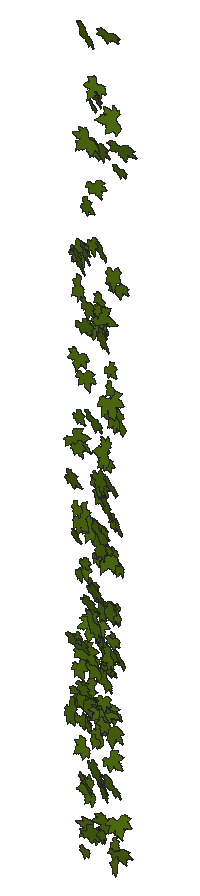
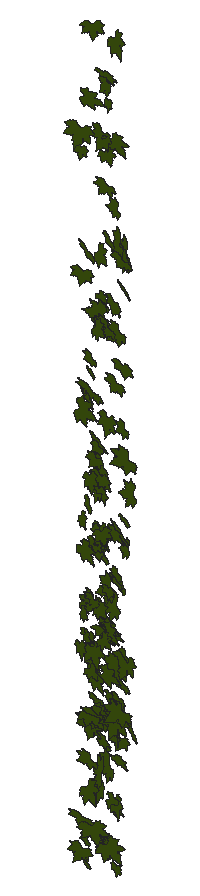
# SketchUp Ruby script. Lengths in inches.
U = 1.inch
M = Sketchup.active_model
def pt(a) = Geom::Point3d.new(a.map { |v| v * U })
def face(e, loops, mat)
  f = e.add_face(loops[0].map { |a| pt(a) })
  loops[1..].each { |l| e.add_face(l.map { |a| pt(a) }).erase! }
  f.material = f.back_material = mat if mat
  f
end
# faces: each face lists its corners as indices into pts; further lists are holes
def faces(e, pts, list, mat = nil) = list.each { |f| face(e, (f[0].is_a?(Array) ? f : [f]).map { |l| l.map { |i| pts[i] } }, mat) }
# xy, xz, yz: faces in a plane at the given z, y or x. An outline is a flat list of corners, or four numbers for a rectangle; further outlines are holes
def ring(l) = l.size == 4 ? [[l[0], l[1]], [l[2], l[1]], [l[2], l[3]], [l[0], l[3]]] : l.each_slice(2).to_a
def flat(e, list, mat, &to3) = list.each { |f| face(e, (f[0].is_a?(Array) ? f : [f]).map { |l| ring(l).map { |u, v| to3.(u, v) } }, mat) }
def xy(e, z, list, mat = nil) = flat(e, list, mat) { |x, y| [x, y, z] }
def xz(e, y, list, mat = nil) = flat(e, list, mat) { |x, z| [x, y, z] }
def yz(e, x, list, mat = nil) = flat(e, list, mat) { |y, z| [x, y, z] }
def lines(e, pts, list) = list.each { |a, b| e.add_line(pt(pts[a]), pt(pts[b])) }
# prism: a flat outline (further loops are holes) pulled along v
def prism(e, loops, v, mat = nil)
  f = face(e, loops, mat); d = Geom::Vector3d.new(v.map { |x| x * U })
  f.pushpull(f.normal.samedirection?(d) ? d.length : -d.length)
end
def box(e, o, s, mat = nil) = prism(e, [[o, [o[0] + s[0], o[1], o[2]], [o[0] + s[0], o[1] + s[1], o[2]], [o[0], o[1] + s[1], o[2]]]], [0, 0, s[2]], mat)
def at(x, y, z, deg = 0) = Geom::Transformation.translation(pt([x, y, z])) * Geom::Transformation.rotation(ORIGIN, Z_AXIS, deg.degrees)
def axes(o, x, y, z) = Geom::Transformation.new([*x, 0, *y, 0, *z, 0, *pt(o).to_a, 1])
def part(name) = M.definitions.add(name)
# library, detail: a bought-in or finely detailed component or shape, given as its bounding box
def library(name, o, s) = part(name).tap { |d| box(d.entities, o, s) }
def detail(e, o, s) = box(e.add_group.entities, o, s)
def put(e, d, t, mat = nil) = e.add_instance(d, t).tap { |i| i.material = mat if mat }
def group(e, t, mat = nil) = e.add_group.tap { |g| g.transformation = t; g.material = mat if mat }.entities
root = M.entities
M.materials.add("[Vegetation Blur 03]").color = [83, 114, 18]
c1 = part("ivy")
xy(c1.entities,0,[[0.782,0,0.786,0,0.787,0.005,0.789,0.009,0.821,0.072,0.875,0.147,1.001,0.272,1.073,0.331,1.137,0.363,1.178,0.379,1.223,0.384,1.272,0.383,1.311,0.374,1.36,0.355,1.399,0.334,1.491,0.285,1.541,0.244,1.583,0.199,1.617,0.15,1.64,0.128,1.662,0.115,1.717,0.105,1.745,0.093,1.784,0.054,1.819,0.057,1.854,0.064,1.882,0.075,1.896,0.074,1.91,0.071,1.937,0.063,1.964,0.053,1.99,0.038,2.016,0.015,2.034,0.002,2.04,0,2.038,0.003,2.036,0.007,2.033,0.038,2.036,0.068,2.045,0.1,2.055,0.116,2.064,0.123,2.077,0.129,2.088,0.129,2.106,0.132,2.118,0.13,2.179,0.132,2.207,0.133,2.225,0.133,2.242,0.138,2.22,0.162,2.207,0.186,2.206,0.213,2.212,0.236,2.228,0.262,2.247,0.274,2.298,0.283,2.355,0.294,2.37,0.296,2.376,0.295,2.377,0.3,2.377,0.303,2.385,0.329,2.411,0.37,2.426,0.392,2.449,0.407,2.511,0.426,2.561,0.444,2.619,0.466,2.589,0.469,2.561,0.476,2.501,0.5,2.449,0.516,2.424,0.523,2.401,0.535,2.377,0.556,2.372,0.568,2.36,0.575,2.268,0.586,2.225,0.592,2.207,0.599,2.194,0.61,2.143,0.65,2.13,0.664,2.122,0.682,2.123,0.7,2.13,0.719,2.148,0.75,2.17,0.781,2.195,0.807,2.221,0.828,2.284,0.874,2.291,0.88,2.288,0.887,2.276,0.9,2.267,0.916,2.265,0.933,2.273,0.967,2.292,1.002,2.313,1.03,2.334,1.054,2.348,1.067,2.358,1.074,2.363,1.076,2.362,1.081,2.35,1.094,2.347,1.11,2.35,1.143,2.359,1.18,2.385,1.254,2.415,1.324,2.448,1.393,2.45,1.4,2.446,1.398,2.44,1.394,2.427,1.383,2.402,1.36,2.376,1.339,2.345,1.324,2.305,1.309,2.282,1.303,2.273,1.306,2.245,1.294,2.212,1.287,2.187,1.291,2.163,1.301,2.142,1.316,2.134,1.327,2.124,1.325,2.09,1.292,2.053,1.259,2.014,1.234,1.973,1.215,1.954,1.21,1.931,1.208,1.909,1.212,1.893,1.22,1.879,1.233,1.872,1.248,1.867,1.281,1.864,1.319,1.821,1.258,1.773,1.197,1.726,1.141,1.698,1.121,1.679,1.116,1.666,1.117,1.647,1.122,1.632,1.129,1.62,1.141,1.617,1.154,1.617,1.219,1.621,1.254,1.623,1.268,1.623,1.281,1.618,1.314,1.606,1.346,1.603,1.375,1.607,1.403,1.603,1.467,1.599,1.499,1.605,1.525,1.614,1.552,1.629,1.577,1.635,1.589,1.629,1.587,1.618,1.582,1.596,1.566,1.581,1.556,1.568,1.552,1.557,1.55,1.545,1.553,1.531,1.562,1.522,1.572,1.504,1.591,1.486,1.611,1.474,1.631,1.457,1.666,1.455,1.684,1.457,1.698,1.452,1.715,1.444,1.728,1.424,1.754,1.419,1.772,1.423,1.786,1.434,1.819,1.444,1.848,1.446,1.855,1.44,1.861,1.43,1.867,1.386,1.904,1.349,1.948,1.326,1.973,1.31,1.995,1.288,2.048,1.284,2.153,1.287,2.254,1.284,2.255,1.282,2.253,1.278,2.247,1.274,2.237,1.266,2.216,1.226,2.125,1.208,2.076,1.184,2.033,1.155,1.984,1.135,1.942,1.111,1.899,1.083,1.861,1.053,1.85,1.059,1.83,1.061,1.809,1.056,1.79,1.049,1.767,1.04,1.749,1.018,1.733,0.994,1.726,0.942,1.734,0.95,1.6875,0.944,1.645,0.932,1.608,0.911,1.585,0.881,1.58,0.854,1.582,0.828,1.588,0.785,1.618,0.773,1.625,0.775,1.614,0.779,1.598,0.796,1.502,0.818,1.402,0.861,1.283,0.882,1.224,0.894,1.174,0.892,1.148,0.886,1.123,0.881,1.107,0.872,1.099,0.849,1.094,0.818,1.092,0.789,1.098,0.762,1.107,0.753,1.113,0.721,1.139,0.698,1.163,0.678,1.194,0.665,1.224,0.628,1.28,0.612,1.312,0.606,1.327,0.606,1.314,0.599,1.282,0.594,1.267,0.581,1.256,0.544,1.245,0.512,1.244,0.473,1.249,0.444,1.256,0.382,1.288,0.339,1.306,0.324,1.316,0.317,1.324,0.309,1.326,0.27,1.314,0.227,1.313,0.185,1.3125,0.152,1.317,0.122,1.328,0.092,1.345,0.073,1.353,0.079,1.338,0.092,1.308,0.117,1.249,0.13,1.215,0.139,1.164,0.147,1.148,0.157,1.136,0.163,1.122,0.174,1.086,0.177,1.067,0.182,1.054,0.186,1.043,0.191,1.038,0.211,1.028,0.237,1.005,0.25,0.974,0.253,0.96,0.25,0.944,0.242,0.914,0.243,0.906,0.249,0.902,0.26,0.894,0.289,0.88,0.307,0.873,0.322,0.862,0.364,0.799,0.403,0.738,0.431,0.709,0.439,0.691,0.441,0.678,0.4375,0.66,0.428,0.645,0.394,0.623,0.303,0.594,0.255,0.581,0.214,0.577,0.179,0.573,0.173,0.568,0.175,0.561,0.167,0.55,0.141,0.523,0.113,0.503,0.077,0.49,0.045,0.486,0.026,0.485,0.019,0.486,0.011,0.483,0,0.471,0.014,0.467,0.044,0.455,0.058,0.447,0.07,0.438,0.097,0.411,0.125,0.394,0.158,0.377,0.174,0.366,0.182,0.359,0.185,0.361,0.242,0.331,0.253,0.316,0.258,0.303,0.262,0.283,0.274,0.278,0.308,0.274,0.341,0.252,0.366,0.226,0.366,0.222,0.37,0.22,0.38,0.221,0.395,0.221,0.425,0.216,0.45,0.207,0.465,0.192,0.473,0.178,0.484,0.15,0.489,0.116,0.483,0.089,0.468,0.058,0.45,0.035,0.435,0.018,0.429,0.011,0.434,0.012,0.438,0.014,0.469,0.019,0.542,0.016,0.581,0.015,0.612,0.027,0.68,0.055,0.696,0.057,0.712,0.052,0.73,0.045,0.741,0.036,0.766,0.014]])
put(root,c1,axes([125.92,173.8,17.01],[0.64437,-0.16461,0.01325],[0.02704,0.17964,-0.52482],[-0.07702,-1.31419,-0.0734]),"[Vegetation Blur 03]")
put(root,c1,axes([125.97,173.8,24.94],[0.20255,-0.18759,0.41357],[0.50926,-0.09194,-0.17269],[-0.07578,-1.11921,-0.05513]),"[Vegetation Blur 03]")
put(root,c1,axes([125.89,173.8,12.75],[0.26152,-0.04302,0.44662],[0.5117,-0.42542,-0.20602],[-0.19512,-1.17335,0.05832]),"[Vegetation Blur 03]")
put(root,c1,axes([125.77,173.8,26.86],[0.3615,0.01419,0.44771],[0.54841,0.02846,-0.29509],[0.01534,-1.35164,-0.00151]),"[Vegetation Blur 03]")
put(root,c1,axes([126.91,173.8,49.39],[0.37946,-0.0754,-0.40939],[-0.47883,0.34147,-0.30552],[-0.15388,-1.24846,-0.05884]),"[Vegetation Blur 03]")
put(root,c1,axes([126.54,173.8,24.12],[0.34373,-0.18323,-0.04475],[-0.06771,-0.09451,-0.28552],[-0.07969,-0.71,0.04955]),"[Vegetation Blur 03]")
put(root,c1,axes([126.41,173.8,16.84],[0.19414,-0.08015,0.20136],[0.24242,-0.09451,-0.1616],[-0.0602,-0.6391,-0.00136]),"[Vegetation Blur 03]")
put(root,c1,axes([126.27,173.8,32.1],[0.54066,-0.11979,-0.01485],[-0.02304,-0.09186,-0.44216],[-0.05647,-1.10941,0.03821]),"[Vegetation Blur 03]")
put(root,c1,axes([126.25,173.8,26.84],[0.30004,-0.03578,0.23182],[0.28092,-0.09842,-0.24458],[-0.04545,-0.84451,0.01868]),"[Vegetation Blur 03]")
put(root,c1,axes([126.29,173.8,12.78],[0.44477,-0.01678,0.0841],[0.10333,0.04659,-0.36253],[-0.00282,-0.93833,-0.0195]),"[Vegetation Blur 03]")
put(root,c1,axes([126.4,173.8,22.17],[0.15681,-0.19135,0.27864],[0.34217,-0.11382,-0.14055],[-0.09017,-0.7647,-0.0488]),"[Vegetation Blur 03]")
put(root,c1,axes([126.36,173.8,28.4375],[0.23733,-0.08095,0.26556],[0.32364,-0.07275,-0.19614],[-0.05179,-0.82556,-0.00876]),"[Vegetation Blur 03]")
put(root,c1,axes([126.15,173.8,37.21],[0.44354,0.00148,0.25414],[0.30752,-0.17731,-0.35733],[-0.04893,-1.101,0.05789]),"[Vegetation Blur 03]")
put(root,c1,axes([126.9,173.8,9.88],[0.41747,-0.18159,-0.28175],[-0.32214,0.27535,-0.34584],[-0.15229,-1.08022,-0.04079]),"[Vegetation Blur 03]")
put(root,c1,axes([126.57,173.8,20.32],[0.21446,-0.11197,0.17329],[0.20462,-0.11686,-0.18055],[-0.07858,-0.60992,0.00278]),"[Vegetation Blur 03]")
put(root,c1,axes([126.19,173.8,37.11],[0.28904,-0.06987,0.39444],[0.46239,-0.30604,-0.23421],[-0.14468,-1.11768,0.03947]),"[Vegetation Blur 03]")
put(root,c1,axes([126.82,173.8,36.16],[0.42016,-0.3703,-0.17602],[-0.23818,-0.04638,-0.36333],[-0.14889,-0.97076,0.0845]),"[Vegetation Blur 03]")
put(root,c1,axes([126.06,173.8,13.94],[0.46309,-0.00814,0.32802],[0.3991,0.15897,-0.37467],[0.04767,-1.25175,-0.04972]),"[Vegetation Blur 03]")
put(root,c1,axes([126.31,173.8,15.31],[0.35031,-0.0224,0.27157],[0.32357,-0.21117,-0.28075],[-0.0784,-0.97156,0.05476]),"[Vegetation Blur 03]")
put(root,c1,axes([127.02,173.8,11.9],[0.35443,-0.19304,-0.2419],[-0.30587,-0.0509,-0.29211],[-0.05567,-0.94941,0.06485]),"[Vegetation Blur 03]")
put(root,c1,axes([126.98,173.8,43.99],[0.532,-0.08529,-0.32199],[-0.3962,-0.04622,-0.4341],[-0.01987,-1.36215,0.03489]),"[Vegetation Blur 03]")
put(root,c1,axes([126.33,173.8,22.68],[0.16553,0.17765,0.51158],[0.60894,-0.40708,-0.109],[-0.17196,-1.2705,0.10646]),"[Vegetation Blur 03]")
put(root,c1,axes([127.1,173.8,13.0625],[0.30175,-0.15566,-0.18852],[-0.22184,0.13329,-0.25383],[-0.09933,-0.77056,-0.00582]),"[Vegetation Blur 03]")
put(root,c1,axes([126.62,173.8,13.79],[0.24227,-0.06001,0.24324],[0.27574,-0.26297,-0.19314],[-0.11679,-0.74533,0.04856]),"[Vegetation Blur 03]")
put(root,c1,axes([127.59,173.8,9.9],[0.23881,-0.20013,-0.4704],[-0.57401,0.16163,-0.20491],[-0.11037,-1.27363,0.04791]),"[Vegetation Blur 03]")
put(root,c1,axes([126.85,173.8,6.07],[0.31854,-0.11206,-0.01065],[-0.01233,0.01101,-0.26373],[-0.05462,-0.65595,-0.00261]),"[Vegetation Blur 03]")
put(root,c1,axes([126.29,173.8,13.81],[0.67064,-0.03297,0.06761],[0.08405,0.14038,-0.54453],[-0.00745,-1.38343,-0.05687]),"[Vegetation Blur 03]")
put(root,c1,axes([126.63,173.8,14.65],[0.43055,-0.17357,0.04955],[0.0586,-0.03425,-0.35804],[-0.08583,-0.8941,0.0041]),"[Vegetation Blur 03]")
put(root,c1,axes([127.21,173.8,7.68],[0.46314,0.05825,-0.39602],[-0.48604,0.04033,-0.37767],[0.00535,-1.37976,-0.02776]),"[Vegetation Blur 03]")
put(root,c1,axes([126.77,173.8,20.93],[0.24085,-0.07286,0.19486],[0.23769,-0.04913,-0.19858],[-0.04198,-0.69616,-0.00638]),"[Vegetation Blur 03]")
put(root,c1,axes([127.5,173.8,23.6875],[0.31165,-0.23246,-0.38206],[-0.4746,0.04633,-0.26229],[-0.08166,-1.15634,0.0663]),"[Vegetation Blur 03]")
put(root,c1,axes([126.45,173.8,33.35],[0.40049,-0.10291,0.28569],[0.35224,0.02026,-0.32774],[-0.03114,-1.09438,-0.03293]),"[Vegetation Blur 03]")
put(root,c1,axes([127.72,173.8,18.65],[0.20411,-0.06117,-0.44075],[-0.53473,0.15542,-0.16833],[-0.08116,-1.17781,0.00068]),"[Vegetation Blur 03]")
put(root,c1,axes([126.75,173.8,20.47],[0.2517,0.01272,0.24338],[0.28699,-0.2291,-0.19581],[-0.08127,-0.76965,0.06231]),"[Vegetation Blur 03]")
put(root,c1,axes([126.33,173.8,37.12],[0.43009,-0.41994,0.38446],[0.46829,-0.19735,-0.38284],[-0.21039,-1.29771,-0.06619]),"[Vegetation Blur 03]")
put(root,c1,axes([126.54,173.8,30.8],[0.46612,-0.06322,0.21313],[0.25778,-0.10592,-0.38046],[-0.05188,-1.09436,0.02451]),"[Vegetation Blur 03]")
put(root,c1,axes([126.33,173.8,15.9375],[0.4004,-0.01607,0.44585],[0.54595,-0.04146,-0.32681],[-0.02086,-1.39316,0.00458]),"[Vegetation Blur 03]")
put(root,c1,axes([127.8,173.8,15.05],[0.07522,-0.13511,-0.31021],[-0.37954,0.11629,-0.06927],[-0.06884,-0.78881,0.04292]),"[Vegetation Blur 03]")
put(root,c1,axes([127.96,173.8,16.33],[0.13923,-0.07198,-0.4584],[-0.56199,0.04465,-0.11479],[-0.02951,-1.18996,0.02342]),"[Vegetation Blur 03]")
put(root,c1,axes([127.37,173.8,43.09],[0.32097,0.04197,-0.19874],[-0.24426,0.07998,-0.2601],[-0.00735,-0.82521,-0.03532]),"[Vegetation Blur 03]")
put(root,c1,axes([126.89,173.8,39.48],[0.11949,-0.05949,0.35767],[0.43416,-0.12523,-0.09989],[-0.06637,-0.92633,-0.00946]),"[Vegetation Blur 03]")
put(root,c1,axes([127.76,173.8,18.05],[0.16976,0.07158,-0.29867],[-0.3654,0.12339,-0.13369],[-0.04012,-0.82092,-0.04613]),"[Vegetation Blur 03]")
put(root,c1,axes([126.89,173.8,34.96],[0.51145,-0.25079,0.06105],[0.06998,-0.0596,-0.42899],[-0.12471,-1.06199,0.00966]),"[Vegetation Blur 03]")
put(root,c1,axes([127.4,173.8,45.46],[0.26677,-0.13263,-0.08131],[-0.08808,0.11667,-0.22242],[-0.07951,-0.57427,-0.02641]),"[Vegetation Blur 03]")
put(root,c1,axes([126.72,173.8,37.63],[0.38011,-0.35457,0.334],[0.40396,-0.18413,-0.33696],[-0.18436,-1.13452,-0.04969]),"[Vegetation Blur 03]")
put(root,c1,axes([127.28,173.8,20.28],[0.33233,-0.0945,-0.02615],[-0.02986,0.03657,-0.27359],[-0.04737,-0.68607,-0.01098]),"[Vegetation Blur 03]")
put(root,c1,axes([128,173.8,38.07],[0.15729,0.04975,-0.38701],[-0.46067,0.26502,-0.11935],[-0.11503,-0.99334,-0.05122]),"[Vegetation Blur 03]")
put(root,c1,axes([127.31,173.8,18.71],[0.56265,-0.26157,-0.25412],[-0.30853,0.09554,-0.47049],[-0.13384,-1.31983,0.01631]),"[Vegetation Blur 03]")
put(root,c1,axes([127.51,173.8,23.48],[0.35115,0.05857,-0.18722],[-0.23024,0.1649,-0.27952],[-0.02054,-0.84722,-0.06735]),"[Vegetation Blur 03]")
put(root,c1,axes([126.87,173.8,6.55],[0.26007,-0.08689,0.38147],[0.46915,0.07766,-0.21026],[0.0126,-1.09796,-0.04506]),"[Vegetation Blur 03]")
put(root,c1,axes([126.98,173.8,18.27],[0.61939,0.05734,-0.0417],[-0.04546,-0.22498,-0.49845],[0.03634,-1.25897,0.08717]),"[Vegetation Blur 03]")
put(root,c1,axes([127.125,173.8,17.87],[0.12985,0.03067,0.35023],[0.42444,-0.14892,-0.10276],[-0.06505,-0.91052,0.02861]),"[Vegetation Blur 03]")
put(root,c1,axes([127.92,173.8,19.54],[0.17674,0.08976,-0.26223],[-0.3229,0.11764,-0.13863],[-0.02967,-0.7454,-0.05345]),"[Vegetation Blur 03]")
put(root,c1,axes([127.11,173.8,29.13],[0.58072,-0.2362,-0.06513],[-0.0644,0.17074,-0.47989],[-0.12408,-1.1941,-0.05574]),"[Vegetation Blur 03]")
put(root,c1,axes([126.87,173.8,18.92],[0.32867,-0.28906,0.36046],[0.45664,0.0115,-0.27589],[-0.07923,-1.13284,-0.09478]),"[Vegetation Blur 03]")
put(root,c1,axes([128.2,173.8,34.0625],[0.08767,0.08949,-0.34433],[-0.41588,0.19217,-0.06267],[-0.08326,-0.86566,-0.04951]),"[Vegetation Blur 03]")
put(root,c1,axes([127.84,173.8,18.08],[0.25432,-0.19046,-0.24423],[-0.28944,0.16036,-0.22043],[-0.11975,-0.79207,0.0141]),"[Vegetation Blur 03]")
put(root,c1,axes([127.08,173.8,40.9],[0.40459,0.02303,0.19859],[0.2435,-0.01333,-0.3302],[0.00625,-0.97145,0.00924]),"[Vegetation Blur 03]")
put(root,c1,axes([127.22,173.8,37.91],[0.28926,-0.09005,0.2261],[0.2622,-0.20395,-0.23621],[-0.09958,-0.79857,0.03483]),"[Vegetation Blur 03]")
put(root,c1,axes([128.27,173.8,12.75],[0.10121,-0.15146,-0.36108],[-0.44341,0.10659,-0.08981],[-0.06746,-0.92784,0.04863]),"[Vegetation Blur 03]")
put(root,c1,axes([127.6,173.8,12.16],[0.30014,-0.14068,-0.03498],[-0.05049,-0.06238,-0.24906],[-0.06295,-0.62077,0.03295]),"[Vegetation Blur 03]")
put(root,c1,axes([127.98,173.8,35.5],[0.20022,-0.05357,-0.19807],[-0.24233,0.03356,-0.1646],[-0.02917,-0.64656,0.00787]),"[Vegetation Blur 03]")
put(root,c1,axes([128.29,173.8,14.2],[0.11196,0.05174,-0.31654],[-0.38834,-0.01941,-0.09199],[0.01605,-0.83049,-0.01757]),"[Vegetation Blur 03]")
put(root,c1,axes([127.5,173.8,46.85],[0.51677,-0.16,-0.11108],[-0.14975,-0.2188,-0.41446],[-0.04632,-1.0777,0.10064]),"[Vegetation Blur 03]")
put(root,c1,axes([127.05,173.8,33.24],[0.28098,0.0713,0.44477],[0.5442,-0.14112,-0.22543],[-0.04527,-1.25382,0.05067]),"[Vegetation Blur 03]")
put(root,c1,axes([127.54,173.8,34.61],[0.25172,-0.04798,0.1294],[0.15152,-0.12662,-0.20371],[-0.0522,-0.59895,0.0327]),"[Vegetation Blur 03]")
put(root,c1,axes([127.64,173.8,23.53],[0.559,-0.25408,-0.226],[-0.26774,0.14716,-0.46713],[-0.14227,-1.27524,-0.00888]),"[Vegetation Blur 03]")
put(root,c1,axes([127.55,173.8,21.52],[0.23635,-0.06465,0.19523],[0.22776,-0.16748,-0.19239],[-0.07957,-0.67142,0.02919]),"[Vegetation Blur 03]")
put(root,c1,axes([127.82,173.8,25.35],[0.41365,-0.19736,-0.16762],[-0.20533,0.04633,-0.34609],[-0.09602,-0.94924,0.01796]),"[Vegetation Blur 03]")
put(root,c1,axes([127.38,173.8,46.01],[0.40968,-0.27629,0.16507],[0.21084,0.00024,-0.34848],[-0.12034,-0.94019,-0.0486]),"[Vegetation Blur 03]")
put(root,c1,axes([127.58,173.8,12.81],[0.09158,0.04301,0.34718],[0.42504,-0.06647,-0.07338],[-0.02723,-0.89296,0.02219]),"[Vegetation Blur 03]")
put(root,c1,axes([128.23,173.8,15.93],[0.35185,-0.14327,-0.37157],[-0.44566,0.19161,-0.29272],[-0.11623,-1.16844,-0.00244]),"[Vegetation Blur 03]")
put(root,c1,axes([127.2,173.8,19.6875],[0.38346,-0.30784,0.36497],[0.45646,-0.05536,-0.32679],[-0.11835,-1.21097,-0.07784]),"[Vegetation Blur 03]")
put(root,c1,axes([127.48,173.8,25.91],[0.59559,-0.20487,-0.02237],[-0.02751,0.00349,-0.49282],[-0.09953,-1.2269,0.00233]),"[Vegetation Blur 03]")
put(root,c1,axes([128.09,173.8,14.13],[0.45581,0.11699,-0.31525],[-0.38742,-0.0162,-0.37405],[0.04848,-1.22937,-0.02507]),"[Vegetation Blur 03]")
put(root,c1,axes([127.34,173.8,43.49],[0.6079,-0.24736,0.08777],[0.11732,0.08596,-0.50313],[-0.11068,-1.26744,-0.05125]),"[Vegetation Blur 03]")
put(root,c1,axes([127.67,173.8,22.82],[0.56324,-0.31646,-0.09717],[-0.11977,0.02711,-0.47626],[-0.15324,-1.18433,0.01506]),"[Vegetation Blur 03]")
put(root,c1,axes([127.73,173.8,17.51],[0.3306,-0.20851,0.08999],[0.10594,-0.063,-0.2822],[-0.10584,-0.71438,-0.00138]),"[Vegetation Blur 03]")
put(root,c1,axes([127.22,173.8,10.5],[0.44878,-0.3413,0.36007],[0.4395,-0.14984,-0.38721],[-0.17027,-1.28634,-0.05043]),"[Vegetation Blur 03]")
put(root,c1,axes([127.98,173.8,17.4],[0.54219,-0.07189,-0.27942],[-0.3337,0.21166,-0.43986],[-0.08416,-1.30245,-0.05606]),"[Vegetation Blur 03]")
put(root,c1,axes([127.85,173.8,49.41],[0.46012,0.08661,-0.09796],[-0.12471,0.12465,-0.37281],[0.02504,-0.97055,-0.05662]),"[Vegetation Blur 03]")
put(root,c1,axes([127.82,173.8,8.16],[0.58678,0.063,-0.19417],[-0.23912,0.05083,-0.47872],[0.01906,-1.30195,-0.02809]),"[Vegetation Blur 03]")
put(root,c1,axes([127.77,173.8,7.27],[0.34382,-0.15266,0.07768],[0.0934,-0.03785,-0.28706],[-0.07642,-0.73315,-0.00136]),"[Vegetation Blur 03]")
put(root,c1,axes([127.33,173.8,13.53],[0.59488,0.11123,0.16598],[0.20655,-0.0688,-0.48585],[0.04022,-1.29188,0.04016]),"[Vegetation Blur 03]")
put(root,c1,axes([127.8,173.8,10.05],[0.51362,-0.33546,-0.11294],[-0.11227,0.20752,-0.43703],[-0.18199,-1.07476,-0.04914]),"[Vegetation Blur 03]")
put(root,c1,axes([128.37,173.8,16.17],[0.24584,0.04332,-0.24097],[-0.29547,0.08344,-0.19842],[-0.01781,-0.78621,-0.03434]),"[Vegetation Blur 03]")
put(root,c1,axes([128.71,173.8,28.09],[0.21833,-0.37386,-0.44692],[-0.55988,0.15366,-0.2024],[-0.13932,-1.20335,0.113]),"[Vegetation Blur 03]")
put(root,c1,axes([128.46,173.8,10.26],[0.33588,0.02262,-0.39753],[-0.47681,0.26549,-0.26596],[-0.10014,-1.18823,-0.067]),"[Vegetation Blur 03]")
put(root,c1,axes([127.51,173.8,33.59],[0.09221,0.01276,0.54145],[0.66339,-0.02223,-0.07517],[-0.00985,-1.37816,0.00623]),"[Vegetation Blur 03]")
put(root,c1,axes([127.8,173.8,27.17],[0.25,-0.03131,0.17773],[0.21716,-0.03407,-0.2044],[-0.02234,-0.68141,0.00205]),"[Vegetation Blur 03]")
put(root,c1,axes([127.77,173.8,18.53],[0.13511,-0.04438,0.35866],[0.42367,-0.24214,-0.11102],[-0.11873,-0.91459,0.01199]),"[Vegetation Blur 03]")
put(root,c1,axes([128.01,173.8,13.24],[0.37736,-0.14693,-0.03133],[-0.04655,-0.08489,-0.31089],[-0.06637,-0.77592,0.03994]),"[Vegetation Blur 03]")
put(root,c1,axes([127.84,173.8,14.22],[0.36114,-0.04689,0.10699],[0.12628,-0.12494,-0.29255],[-0.0419,-0.78067,0.04039]),"[Vegetation Blur 03]")
put(root,c1,axes([128.24,173.8,16.5625],[0.39633,-0.13888,-0.234],[-0.27566,0.17367,-0.32719],[-0.1038,-0.99151,-0.02453]),"[Vegetation Blur 03]")
put(root,c1,axes([127.99,173.8,22.66],[0.10493,-0.03643,0.24088],[0.29195,-0.08918,-0.08683],[-0.04677,-0.63839,-0.00162]),"[Vegetation Blur 03]")
put(root,c1,axes([127.82,173.8,26.63],[0.3534,-0.02851,0.14206],[0.17452,0.03242,-0.28817],[-0.00545,-0.81,-0.01653]),"[Vegetation Blur 03]")
put(root,c1,axes([127.96,173.8,22.42],[0.40755,-0.11351,-0.00014],[0.00098,0.01751,-0.33557],[-0.05515,-0.83847,-0.00699]),"[Vegetation Blur 03]")
put(root,c1,axes([128.27,173.8,26.03],[0.4235,-0.13743,-0.21645],[-0.24668,0.24247,-0.3457],[-0.1181,-0.99928,-0.05411]),"[Vegetation Blur 03]")
put(root,c1,axes([128.04,173.8,15.86],[0.26031,-0.0805,0.12545],[0.1556,0.01165,-0.21388],[-0.03078,-0.62197,-0.02024]),"[Vegetation Blur 03]")
put(root,c1,axes([127.52,173.8,25.87],[0.47957,-0.26061,0.31785],[0.37221,-0.23733,-0.40467],[-0.1708,-1.24893,0.01057]),"[Vegetation Blur 03]")
put(root,c1,axes([127.91,173.8,19.28],[0.41549,-0.08208,0.11963],[0.15106,0.12998,-0.33542],[-0.01613,-0.89729,-0.05953]),"[Vegetation Blur 03]")
put(root,c1,axes([128.57,173.8,17.2],[0.33509,-0.2609,-0.26753],[-0.3303,0.08476,-0.28857],[-0.12012,-0.96089,0.04719]),"[Vegetation Blur 03]")
put(root,c1,axes([128.9,173.8,17.78],[0.07952,-0.02515,-0.25316],[-0.29832,0.17612,-0.06516],[-0.08589,-0.63499,-0.00805]),"[Vegetation Blur 03]")
put(root,c1,axes([128.02,173.8,22.26],[0.59751,-0.1415,-0.08723],[-0.11552,-0.16395,-0.48523],[-0.05298,-1.23827,0.07421]),"[Vegetation Blur 03]")
put(root,c1,axes([129.14,173.8,45.66],[0.17867,-0.14742,-0.47769],[-0.58909,-0.10072,-0.14187],[0.02629,-1.25528,0.06748]),"[Vegetation Blur 03]")
put(root,c1,axes([129.32,173.8,29.72],[0.10377,0.02186,-0.53621],[-0.65451,0.12482,-0.08356],[-0.05827,-1.36305,-0.01625]),"[Vegetation Blur 03]")
put(root,c1,axes([127.79,173.8,33.17],[0.29678,-0.27186,0.42657],[0.50911,-0.26247,-0.26224],[-0.17731,-1.20867,-0.039]),"[Vegetation Blur 03]")
put(root,c1,axes([129.11,173.8,18.94],[0.04974,-0.00028,-0.27725],[-0.32677,0.19308,-0.03908],[-0.09286,-0.67961,-0.01099]),"[Vegetation Blur 03]")
put(root,c1,axes([129.2,173.8,19.46],[0.08632,-0.07212,-0.36138],[-0.4424,0.06914,-0.07256],[-0.03977,-0.92577,0.02273]),"[Vegetation Blur 03]")
put(root,c1,axes([128.08,173.8,9.62],[0.09448,-0.24372,0.47773],[0.55916,-0.39227,-0.10514],[-0.20978,-1.15536,-0.06508]),"[Vegetation Blur 03]")
put(root,c1,axes([128.88,173.8,22.4375],[0.39881,-0.16855,-0.40776],[-0.49292,0.16963,-0.33214],[-0.11562,-1.30452,0.00949]),"[Vegetation Blur 03]")
put(root,c1,axes([128.21,173.8,31.48],[0.21376,-0.00368,0.2636],[0.3197,-0.11113,-0.17293],[-0.04601,-0.78924,0.02312]),"[Vegetation Blur 03]")
put(root,c1,axes([128.58,173.8,31.12],[0.30532,-0.22387,-0.07925],[-0.10993,-0.04866,-0.26046],[-0.09582,-0.65751,0.04626]),"[Vegetation Blur 03]")
put(root,c1,axes([129.11,173.8,6.12],[0.10497,-0.16799,-0.28426],[-0.34085,0.17977,-0.10055],[-0.10859,-0.72666,0.04084]),"[Vegetation Blur 03]")
put(root,c1,axes([128.375,173.8,17.5625],[0.3425,-0.04443,0.04433],[0.05384,-0.01893,-0.28004],[-0.02276,-0.71335,0.00467]),"[Vegetation Blur 03]")
put(root,c1,axes([127.95,173.8,13.03],[0.66487,-0.12258,0.05657],[0.06821,-0.03171,-0.54475],[-0.06083,-1.37523,0.00752]),"[Vegetation Blur 03]")
put(root,c1,axes([129,173.8,23.85],[0.19183,-0.05588,-0.2698],[-0.31224,0.23474,-0.15552],[-0.11192,-0.75067,-0.02855]),"[Vegetation Blur 03]")
put(root,c1,axes([128,173.8,18.98],[0.40007,-0.13518,0.27607],[0.33165,-0.13835,-0.33079],[-0.0935,-1.06919,0.0079]),"[Vegetation Blur 03]")
put(root,c1,axes([128.08,173.8,10.75],[0.24435,0.09355,0.35761],[0.44053,-0.04867,-0.19849],[0.00137,-1.03125,0.04181]),"[Vegetation Blur 03]")
put(root,c1,axes([127.78,173.8,29.74],[0.49312,0.07516,0.37451],[0.45503,-0.28887,-0.38996],[-0.06962,-1.3557,0.10386]),"[Vegetation Blur 03]")
put(root,c1,axes([127.9375,173.8,24.64],[0.40386,-0.35784,0.38449],[0.46593,-0.19708,-0.35483],[-0.18733,-1.26162,-0.05362]),"[Vegetation Blur 03]")
put(root,c1,axes([128.6,173.8,6.54],[0.09713,0.02395,0.23937],[0.28996,-0.10667,-0.07669],[-0.04564,-0.62678,0.0222]),"[Vegetation Blur 03]")
put(root,c1,axes([128.41,173.8,36.24],[0.48068,0.01776,0.03152],[0.03794,0.06838,-0.39147],[0.01124,-0.98997,-0.02647]),"[Vegetation Blur 03]")
put(root,c1,axes([128.8125,173.8,29.92],[0.4464,-0.35085,-0.18371],[-0.23796,-0.0009,-0.38487],[-0.15203,-1.02878,0.06299]),"[Vegetation Blur 03]")
put(root,c1,axes([128.52,173.8,23.75],[0.21308,-0.12887,0.25392],[0.29486,-0.2048,-0.18116],[-0.11737,-0.74847,0.00585]),"[Vegetation Blur 03]")
put(root,c1,axes([128.39,173.8,6.32],[0.46585,0.02288,0.14137],[0.17091,0.11775,-0.37813],[0.0303,-1.01595,-0.04064]),"[Vegetation Blur 03]")
put(root,c1,axes([128.94,173.8,17.05],[0.36602,-0.17334,-0.17958],[-0.2031,0.19186,-0.30487],[-0.11941,-0.85763,-0.0319]),"[Vegetation Blur 03]")
put(root,c1,axes([128.34,173.8,43.67],[0.63593,0.00439,0.02808],[0.0337,0.19557,-0.51321],[0.00724,-1.29586,-0.07736]),"[Vegetation Blur 03]")
put(root,c1,axes([128.77,173.8,42.55],[0.37054,-0.08411,-0.02834],[-0.02969,0.09383,-0.30232],[-0.04467,-0.76008,-0.03419]),"[Vegetation Blur 03]")
put(root,c1,axes([128.32,173.8,7.84],[0.46596,0.12424,0.22352],[0.28037,-0.18097,-0.37349],[0.00652,-1.09739,0.0869]),"[Vegetation Blur 03]")
put(root,c1,axes([128.36,173.8,36.9],[0.46976,-0.15316,0.21327],[0.23871,-0.28032,-0.3819],[-0.12977,-1.07007,0.06952]),"[Vegetation Blur 03]")
